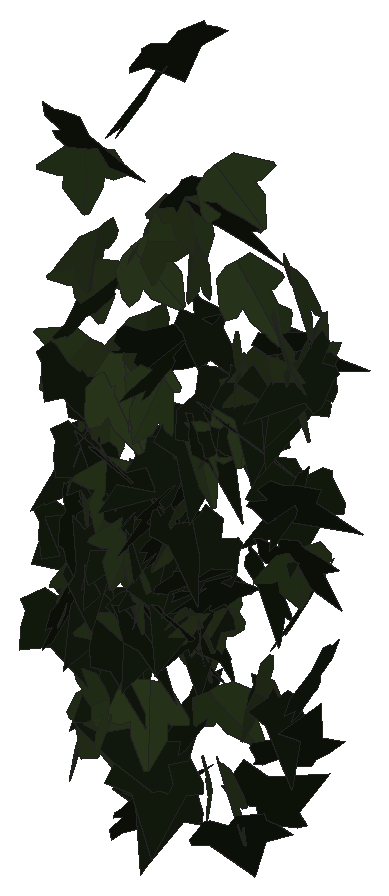
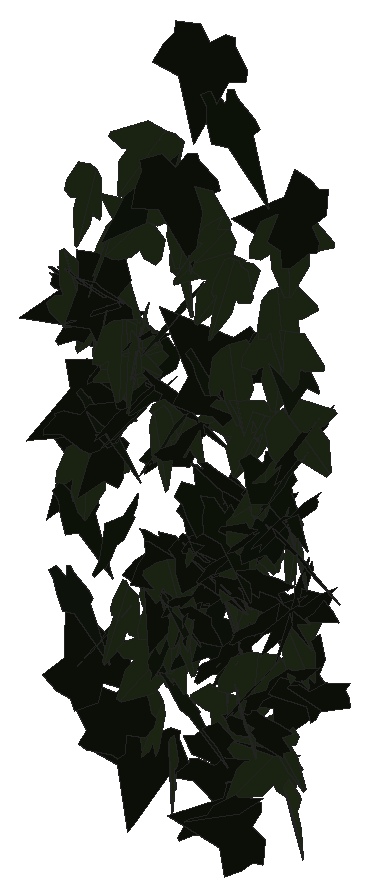
# SketchUp Ruby script. Lengths in inches.
U = 1.inch
M = Sketchup.active_model
def pt(a) = Geom::Point3d.new(a.map { |v| v * U })
def face(e, loops, mat)
  f = e.add_face(loops[0].map { |a| pt(a) })
  loops[1..].each { |l| e.add_face(l.map { |a| pt(a) }).erase! }
  f.material = f.back_material = mat if mat
  f
end
# faces: each face lists its corners as indices into pts; further lists are holes
def faces(e, pts, list, mat = nil) = list.each { |f| face(e, (f[0].is_a?(Array) ? f : [f]).map { |l| l.map { |i| pts[i] } }, mat) }
# xy, xz, yz: faces in a plane at the given z, y or x. An outline is a flat list of corners, or four numbers for a rectangle; further outlines are holes
def ring(l) = l.size == 4 ? [[l[0], l[1]], [l[2], l[1]], [l[2], l[3]], [l[0], l[3]]] : l.each_slice(2).to_a
def flat(e, list, mat, &to3) = list.each { |f| face(e, (f[0].is_a?(Array) ? f : [f]).map { |l| ring(l).map { |u, v| to3.(u, v) } }, mat) }
def xy(e, z, list, mat = nil) = flat(e, list, mat) { |x, y| [x, y, z] }
def xz(e, y, list, mat = nil) = flat(e, list, mat) { |x, z| [x, y, z] }
def yz(e, x, list, mat = nil) = flat(e, list, mat) { |y, z| [x, y, z] }
def lines(e, pts, list) = list.each { |a, b| e.add_line(pt(pts[a]), pt(pts[b])) }
# prism: a flat outline (further loops are holes) pulled along v
def prism(e, loops, v, mat = nil)
  f = face(e, loops, mat); d = Geom::Vector3d.new(v.map { |x| x * U })
  f.pushpull(f.normal.samedirection?(d) ? d.length : -d.length)
end
def box(e, o, s, mat = nil) = prism(e, [[o, [o[0] + s[0], o[1], o[2]], [o[0] + s[0], o[1] + s[1], o[2]], [o[0], o[1] + s[1], o[2]]]], [0, 0, s[2]], mat)
def at(x, y, z, deg = 0) = Geom::Transformation.translation(pt([x, y, z])) * Geom::Transformation.rotation(ORIGIN, Z_AXIS, deg.degrees)
def axes(o, x, y, z) = Geom::Transformation.new([*x, 0, *y, 0, *z, 0, *pt(o).to_a, 1])
def part(name) = M.definitions.add(name)
# library, detail: a bought-in or finely detailed component or shape, given as its bounding box
def library(name, o, s) = part(name).tap { |d| box(d.entities, o, s) }
def detail(e, o, s) = box(e.add_group.entities, o, s)
def put(e, d, t, mat = nil) = e.add_instance(d, t).tap { |i| i.material = mat if mat }
def group(e, t, mat = nil) = e.add_group.tap { |g| g.transformation = t; g.material = mat if mat }.entities
root = M.entities
M.materials.add("efeu1").color = [18, 25, 13]
M.materials.add("efeu2").color = [43, 57, 29]
c1 = part("ivyleaf_9")
p = [[1.54,2.16,1.25],[1.36,2.04,1.19],[-0.21,0.99,0.68],[-0.71,1.11,0.82],[-0.85,0.86,0.67],[-0.8,0.17,0.21],
  [-0.9,-0.01,0.1],[-0.67,-0.16,-0.02],[-0.08,-0.08,-0.05],[-0.03,-0.6,-0.4],[0.65,-0.88,-0.66],[0.83,-0.6,-0.49],
  [1.29,-0.42,-0.43],[1.8125,-0.07,-0.26],[1.21,0.44,0.15]]
faces(c1.entities,p,[[0,1,2,3,4,5,6,7,8,9,10,11,12,13,14]],"efeu1")
c2 = part("ivyleaf_10")
p = [[0,0.5,-0.03],[-0.0625,2.02,-0.43],[-0.19,2.01,-0.46],[-0.54,1.05,-0.29],[-0.52,0.625,-0.18],[-0.83,0.76,-0.28],
  [-1.16,0.64,-0.33],[-1.15,0.33,-0.24],[-0.77,-0.39,0.02],[-0.3,-0.51,0.16],[0.04,-0.48,0.23],[-0.02,2.01,-0.4375],
  [-0.06,2.01,-0.43],[0.04,-0.49,0.23],[0.67,-0.49,0.14],[1.38,0.36,-0.2],[1.375,0.51,-0.24],[0.81,0.65,-0.19],
  [0.62,0.59,-0.15],[0.6,1.09,-0.28],[0.5,1.23,-0.31]]
faces(c2.entities,p,[[0,1,2,3,4,5,6,7,8,9,10],[11,12,0,13,14,15,16,17,18,19,20]],"efeu2")
put(root,c1,axes([557.47,132.86,219.08],[0.60658,-0.54381,0.3875],[0.43826,-0.07075,-0.78533],[0.5038,0.71631,0.21662]))
put(root,c2,axes([552.82,132.8,225.43],[-0.73036,-0.58311,0.05549],[-0.04524,-0.03227,-0.93458],[0.584,-0.73175,-0.003]))
put(root,c2,axes([552.45,133.0625,219.47],[-0.53208,-0.47157,0.54848],[-0.39673,-0.37907,-0.71079],[0.60482,-0.66351,0.01627]))
put(root,c1,axes([554.42,132.75,215.25],[0.17808,-0.1101,0.87837],[-0.72136,0.5013,0.20908],[-0.51313,-0.74294,0.01091]))
put(root,c1,axes([555.13,132.63,228.52],[-0.57807,0.85894,-0.08509],[0.04941,-0.06931,-1.03534],[-0.86173,-0.58018,-0.00229]))
put(root,c1,axes([558.02,132.43,207.03],[0.55639,0.71118,-0.20448],[-0.13118,-0.15698,-0.90294],[-0.72827,0.57161,0.00643]))
put(root,c1,axes([559.49,132.37,217.54],[0.80214,0.25674,0.39294],[0.37203,0.12662,-0.8422],[-0.28619,0.88419,0.00651]))
put(root,c2,axes([557.59,132.82,208.22],[-0.69387,0.55552,-0.2453],[0.17651,-0.17188,-0.88856],[-0.58105,-0.7156,0.023]))
put(root,c2,axes([558.2,132.77,223.7],[0.71979,0.11011,0.65936],[0.63025,0.21122,-0.72329],[-0.22285,0.95301,0.08412]))
put(root,c2,axes([553.01,132.875,223.02],[-0.11838,-0.92552,-0.06851],[0.0011,0.06893,-0.93303],[0.92805,-0.11814,-0.00763]))
put(root,c1,axes([559.84,132.79,217.375],[-0.68343,0.5681,-0.01902],[0.01467,-0.01209,-0.88872],[-0.56823,-0.68359,-0.00008]))
put(root,c1,axes([552.0625,132.87,219.16],[0.36984,-0.75674,-0.35005],[-0.1662,0.30835,-0.84218],[0.81704,0.40527,-0.01286]))
put(root,c2,axes([560.07,132.7,224.38],[-0.82635,0.45852,0.04383],[-0.04635,0.00679,-0.9449],[-0.45827,-0.82749,0.01653]))
put(root,c1,axes([559.76,132.48,216.09],[0.90589,0.26652,-0.11191],[-0.10848,-0.02779,-0.94428],[-0.26794,0.91236,0.00393]))
put(root,c2,axes([556.46,133.02,218.1],[-0.81948,0.13079,-0.38359],[0.30779,-0.36207,-0.781],[-0.26365,-0.82921,0.28052]))
put(root,c2,axes([554.125,132.95,213.34],[-0.68982,0.39589,-0.33862],[0.22406,-0.28179,-0.7859],[-0.47031,-0.71492,0.12226]))
put(root,c2,axes([553.75,133.17,215.97],[-0.44081,-0.72991,0.3487],[-0.07843,-0.35668,-0.84575],[0.80511,-0.43438,0.10853]))
put(root,c1,axes([552.54,133.06,213.79],[-0.46389,-0.57428,-0.502],[0.31988,0.38692,-0.73822],[0.69245,-0.56347,0.00472]))
put(root,c1,axes([551.97,132.91,225.97],[0.66825,-0.28484,0.59393],[0.54404,-0.23831,-0.72641],[0.37135,0.8617,-0.00457]))
put(root,c2,axes([554.13,133.17,214.35],[-0.31867,-0.76691,0.29919],[-0.04618,-0.30366,-0.82757],[0.8219,-0.31441,0.0695]))
put(root,c1,axes([553.24,132.28,221.09],[0.00284,0.77291,0.49877],[-0.27206,0.47716,-0.73788],[-0.87872,-0.14523,0.23006]))
put(root,c2,axes([553.43,132.79,208.18],[-0.73599,-0.15467,-0.52759],[0.5255,0.06129,-0.75104],[0.16165,-0.90348,0.03937]))
put(root,c1,axes([557.26,132.54,225.55],[0.92495,0.13837,-0.00241],[-0.01675,0.09577,-0.93018],[-0.13737,0.91998,0.0972]))
put(root,c2,axes([554.96,132.5,223.23],[0.32845,0.66171,0.55842],[0.18607,0.52935,-0.73671],[-0.84561,0.3735,0.05479]))
put(root,c2,axes([559.94,132.89,215.67],[-0.43488,-0.76847,-0.11966],[0.04324,0.113,-0.88281],[0.77653,-0.43666,-0.01786]))
put(root,c1,axes([555.6,132.93,220.31],[-0.64013,0.64987,-0.10604],[0.00694,-0.14122,-0.90738],[-0.65842,-0.63329,0.09353]))
put(root,c2,axes([554.73,133,209.54],[0.93693,0.16638,0.14697],[0.14195,0.04108,-0.95147],[-0.17068,0.9475,0.01544]))
put(root,c1,axes([554.21,133.17,211.6],[0.49252,-0.69361,0.12402],[0.11232,-0.07209,-0.84926],[0.6956,0.50276,0.04932]))
put(root,c2,axes([554.95,132.99,219.03],[0.84963,-0.22571,-0.25975],[-0.23718,0.11724,-0.87766],[0.24933,0.88068,0.05027]))
put(root,c2,axes([559.14,132.85,221.28],[-0.91001,0.04005,0.01507],[-0.01501,0.00183,-0.91089],[-0.04008,-0.91014,-0.00117]))
put(root,c1,axes([555.9,132.51,230.2],[0.26752,0.91147,-0.06237],[-0.02542,-0.05754,-0.94988],[-0.91324,0.2686,0.00817]))
put(root,c2,axes([553.22,132.78,209.03],[0.49664,-0.30401,-0.70783],[-0.57736,0.41067,-0.58147],[0.51001,0.76094,0.03102]))
put(root,c2,axes([552.15,133.3,212.64],[0.19158,-0.8497,0.28444],[0.08541,-0.27223,-0.87074],[0.89196,0.20857,0.02229]))
put(root,c2,axes([556.31,132.91,225.16],[-0.82074,-0.4387,-0.06342],[0.05426,0.03301,-0.93062],[0.43992,-0.82252,-0.00353]))
put(root,c2,axes([559.48,132.75,222.6],[-0.51977,0.73445,0.16439],[-0.07068,0.15127,-0.89929],[-0.7493,-0.52374,-0.0292]))
put(root,c1,axes([554.99,133.31,207.55],[-0.51264,-0.63793,-0.33703],[0.23677,0.2418,-0.81781],[0.68153,-0.56385,0.0306]))
put(root,c1,axes([555.45,133.23,215.97],[-0.42253,0.57344,-0.53397],[0.13625,-0.54364,-0.69165],[-0.77162,-0.41001,0.17027]))
put(root,c1,axes([560.29,133.34,221.58],[-0.90128,0.04055,0.01997],[-0.02487,-0.11203,-0.89509],[-0.03774,-0.89452,0.11301]))
put(root,c1,axes([555.27,133.27,216.95],[-0.88487,0.07931,0.06994],[-0.07249,-0.02589,-0.88784],[-0.07698,-0.88725,0.03216]))
put(root,c2,axes([553.8,132.83,218.81],[0.55344,0.69538,0.34378],[0.23498,0.25218,-0.88838],[-0.73927,0.60074,-0.02501]))
put(root,c1,axes([555.15,133.2,207.66],[-0.30047,0.08024,0.86489],[-0.85799,0.11523,-0.30876],[-0.13539,-0.90832,0.03723]))
put(root,c1,axes([555.43,133.4,215.14],[0.2952,-0.80922,0.10957],[0.04443,-0.10042,-0.86136],[0.8154,0.29844,0.00727]))
put(root,c1,axes([559.91,133.48,221.53],[-0.7914,-0.35926,-0.22467],[0.25236,-0.01727,-0.86133],[0.34038,-0.8225,0.11622]))
put(root,c2,axes([555.5,132.48,224.08],[0.003,-0.3785,-0.84862],[0.30986,0.80046,-0.35592],[0.87602,-0.28184,0.1288]))
put(root,c2,axes([557.65,132.68,226.58],[0.46737,0.61433,0.53449],[0.19395,0.51455,-0.76101],[-0.79086,0.48923,0.12923]))
put(root,c1,axes([558.19,133.55,219.9],[-0.11464,-0.89674,0.0292],[-0.00024,-0.02941,-0.90403],[0.89721,-0.11459,0.00349]))
put(root,c1,axes([555.5,133.63,213.07],[-0.35716,-0.82388,0.04236],[0.00027,-0.04628,-0.89777],[0.82497,-0.35668,0.01863]))
put(root,c1,axes([553.42,133.36,210.83],[0.32268,-0.82099,-0.07439],[-0.00206,0.07908,-0.88172],[0.82436,0.32156,0.02692]))
put(root,c1,axes([558.76,133.6,210.63],[0.20915,-0.85335,0.22357],[0.09497,-0.20665,-0.87761],[0.87702,0.22588,0.04172]))
put(root,c2,axes([554.46,133.22,220.83],[-0.17141,-0.89668,-0.00621],[0.01263,0.00391,-0.91284],[0.89661,-0.17147,0.01167]))
put(root,c2,axes([555.4,133.72,214.92],[-0.11244,0.3847,-0.77795],[-0.0815,-0.78567,-0.37674],[-0.86404,0.02405,0.13678]))
put(root,c2,axes([558.76,132.67,211.3],[0.06453,-0.59585,-0.75032],[-0.0064,0.75173,-0.59753],[0.95811,0.04515,0.04654]))
put(root,c1,axes([552.05,132.42,211.17],[0.1319,0.30454,0.864],[0.24818,0.82839,-0.32988],[-0.88184,0.27868,0.03639]))
put(root,c1,axes([556.6875,132.99,226.08],[0.03785,0.86944,-0.33901],[-0.00626,-0.33905,-0.87023],[-0.93318,0.03754,-0.00791]))
put(root,c1,axes([554.51,132.99,220.05],[0.74729,0.66545,-0.25331],[0.16861,0.19138,1.00019],[0.69178,-0.7655,0.02986]))
put(root,c1,axes([556.42,133.03,221.75],[0.62156,-0.55565,-0.384],[-0.1649,0.38122,-0.81855],[0.65499,0.62327,0.15832]))
put(root,c2,axes([557.93,133.27,219.65],[0.50584,0.7239,-0.12618],[-0.05878,-0.11283,-0.88298],[-0.73246,0.50898,-0.01628]))
put(root,c2,axes([554.12,133.29,219.375],[0.7918,0.44741,-0.06621],[-0.05021,-0.04571,-0.90934],[-0.44949,0.79325,-0.01505]))
put(root,c1,axes([559.24,133.69,220.67],[-0.41567,-0.78854,-0.01827],[0.00399,0.01855,-0.89137],[0.78874,-0.41566,-0.00512]))
put(root,c1,axes([552.3125,133.33,216.57],[0.27475,-0.80355,-0.27842],[-0.02287,0.2855,-0.84656],[0.85011,0.26738,0.06721]))
put(root,c2,axes([552.73,133.17,221.86],[-0.79276,-0.45023,-0.02683],[0.01665,0.025,-0.91159],[0.45072,-0.79282,-0.01351]))
put(root,c1,axes([555.09,133.02,212.18],[0.89612,-0.10876,-0.00098],[-0.0009,0.00072,-0.9027],[0.10876,0.89612,0.00061]))
put(root,c2,axes([556.39,133.1,223.6875],[-0.68613,0.51321,0.36316],[-0.43244,0.00496,-0.82403],[-0.45637,-0.7763,0.23482]))
put(root,c1,axes([557.08,133.32,219.06],[-0.79787,0.2624,0.30518],[-0.28767,0.10211,-0.83989],[-0.28149,-0.84812,-0.0067]))
put(root,c1,axes([552.2,132.76,214.43],[0.32513,-0.07581,-0.86332],[-0.71821,0.49246,-0.31372],[0.48501,0.78007,0.11416]))
put(root,c1,axes([552.98,133.0625,216.24],[0.89559,-0.12999,-0.0139],[-0.01379,0.00174,-0.90498],[0.13,0.8957,-0.00026]))
put(root,c2,axes([557.19,133.08,210.3125],[-0.71086,-0.23411,-0.49745],[0.46955,0.16444,-0.74837],[0.28598,-0.8519,-0.00776]))
put(root,c2,axes([559.35,133.24,220.93],[-0.68691,0.54402,-0.25399],[0.20789,-0.14656,-0.87614],[-0.56325,-0.71755,-0.01361]))
put(root,c1,axes([556.04,133.77,217.85],[-0.13048,-0.88076,0.08198],[-0.00873,-0.08158,-0.89037],[0.88453,-0.13073,0.00331]))
put(root,c1,axes([552.27,133.5,217.93],[0.4561,-0.77566,-0.00192],[0.01766,0.01262,-0.89956],[0.77546,0.45593,0.02162]))
put(root,c1,axes([551.58,133.38,211.17],[-0.07751,-0.75806,-0.52624],[0.20412,0.50093,-0.75166],[0.89996,-0.17891,0.12516]))
put(root,c1,axes([558.36,133.26,207.48],[-0.0117,-0.16519,0.86926],[0.86455,-0.18713,-0.02392],[0.18829,0.84895,0.16387]))
put(root,c2,axes([554.68,132.99,223.42],[0.0315,-0.75243,-0.5322],[0.12535,0.53106,-0.7434],[0.91306,-0.04694,0.12042]))
put(root,c1,axes([555.47,133.52,216.48],[-0.57404,0.52944,-0.42353],[0.13641,-0.45341,-0.75168],[-0.66414,-0.55074,0.21168]))
put(root,c2,axes([558.35,133.41,220.4],[-0.1264,-0.90194,-0.0052],[0.00448,0.00462,-0.91075],[0.90195,-0.12642,0.0038]))
put(root,c2,axes([552.16,133.4,215.85],[-0.65587,0.57855,-0.19807],[0.0354,-0.25405,-0.85926],[-0.61049,-0.63629,0.16297]))
put(root,c1,axes([553.24,133.27,217.8125],[-0.47573,0.73736,-0.16871],[0.0171,-0.18877,-0.87325],[-0.75622,-0.46814,0.08639]))
put(root,c1,axes([556.41,133.12,213.74],[0.34982,0.70164,-0.38547],[-0.20828,-0.32641,-0.78316],[-0.77298,0.40548,0.03657]))
put(root,c1,axes([560.11,133.33,214.54],[-0.53911,0.67101,-0.2361],[0.15429,-0.17888,-0.86071],[-0.6944,-0.5607,-0.00795]))
put(root,c1,axes([555.36,133.59,213.96],[-0.85781,0.1344,-0.06234],[0.05082,-0.07711,-0.8656],[-0.13917,-0.85661,0.06814]))
put(root,c1,axes([556.37,133.48,212.5625],[-0.70701,0.44443,-0.24847],[0.18721,-0.16849,-0.83407],[-0.47351,-0.73021,0.04123]))
put(root,c1,axes([554.31,133.95,211.65],[-0.26299,-0.79086,0.24415],[-0.08866,-0.22778,-0.83336],[0.82292,-0.27729,-0.01176]))
put(root,c2,axes([552.1875,133.4375,207.5],[0.46432,-0.7013,-0.10271],[-0.05453,0.08708,-0.84108],[0.70668,0.4675,0.00258]))
put(root,c1,axes([555.4,133.54,214.78],[-0.29548,0.60973,-0.55694],[0.12928,-0.55007,-0.6708],[-0.81562,-0.30808,0.09544]))
put(root,c1,axes([556.38,133.67,217.9375],[0.42012,-0.78906,0.09861],[0.05516,-0.08234,-0.89388],[0.79328,0.42361,0.00993]))
put(root,c2,axes([552.04,133.54,216.3],[0.52172,-0.73387,0.02376],[0.01412,-0.01911,-0.90042],[0.73412,0.52191,0.00043]))
put(root,c2,axes([553.1,133.49,217.59],[0.01828,0.8674,-0.26461],[0.00516,-0.26476,-0.86753],[-0.90685,0.01598,-0.01027]))
put(root,c2,axes([554.3,133.53,212.99],[0.52773,-0.68683,-0.0084],[-0.00787,0.00454,-0.86615],[0.68684,0.52777,-0.00347]))
put(root,c1,axes([559.47,133.76,217.54],[-0.42417,-0.75561,-0.222],[0.11379,0.1907,-0.8665],[0.77928,-0.43913,0.00569]))
put(root,c2,axes([553.49,133.38,211.28],[-0.67821,-0.57029,-0.05161],[0.0356,0.03786,-0.88609],[0.57151,-0.67912,-0.00605]))
put(root,c1,axes([558.08,133.97,213.97],[0.23714,-0.66891,0.52929],[0.17067,-0.50105,-0.70968],[0.83574,0.29213,-0.00526]))
put(root,c1,axes([551.69,133.51,213.93],[0.27282,-0.7897,-0.36067],[0.03089,0.38665,-0.82322],[0.86761,0.23456,0.14273]))
put(root,c1,axes([552.375,133.66,216.01],[-0.86087,0.20506,-0.06305],[0.0559,-0.03734,-0.88465],[-0.20712,-0.86237,0.02331]))
put(root,c2,axes([557.85,132.94,220.67],[0.23391,-0.34468,-0.80439],[-0.161,0.80146,-0.39024],[0.86019,0.24373,0.1457]))
put(root,c1,axes([554.01,134.02,215.05],[-0.11401,-0.85111,0.18479],[0.01591,-0.18837,-0.85779],[0.87079,-0.10799,0.03987]))
put(root,c1,axes([556.48,133.84,214.61],[-0.84406,-0.19522,-0.12449],[0.13551,-0.03492,-0.86399],[0.18775,-0.85248,0.0639]))
put(root,c2,axes([556.02,133.4,212.21],[-0.67776,0.5337,-0.11149],[0.08344,-0.07425,-0.86265],[-0.5388,-0.68285,0.00666]))
put(root,c1,axes([559,133.51,209.08],[0.68242,0.57121,0.1933],[-0.14819,-0.12412,0.88994],[0.58454,-0.69833,-0.00005]))
put(root,c1,axes([554.45,133.94,215.48],[-0.48101,-0.73637,-0.10209],[0.09824,0.05757,-0.87811],[0.73689,-0.48835,0.05042]))
put(root,c1,axes([556.3,133.41,209.65],[-0.68908,0.58055,0.11951],[-0.09207,0.07621,-0.90103],[-0.58553,-0.6952,0.00103]))
put(root,c2,axes([556.49,133.55,212.23],[-0.44443,-0.77722,-0.01084],[0.00171,0.01151,-0.8953],[0.77729,-0.44441,-0.00422]))
put(root,c2,axes([555.81,133.6,212.3],[-0.06507,-0.86588,-0.03723],[-0.00407,0.03764,-0.8683],[0.86667,-0.06484,-0.00688]))
put(root,c1,axes([553.42,133.9,209.85],[-0.81513,-0.24427,-0.00506],[0.0047,0.00197,-0.85094],[0.24428,-0.81514,-0.00054]))
put(root,c1,axes([554.62,134.07,206.45],[-0.32464,-0.82684,0.07489],[-0.02001,-0.0726,-0.88826],[0.82999,-0.32516,0.00788]))
put(root,c1,axes([552.82,133.9,213.96],[-0.84381,-0.19726,-0.18221],[0.19112,-0.0191,-0.86443],[0.18864,-0.86305,0.06078]))
put(root,c2,axes([558.66,133.53,220],[0.18126,-0.00387,-0.88794],[-0.86825,0.18906,-0.17806],[0.186,0.88631,0.03411]))
put(root,c1,axes([556.49,133.13,213.36],[0.48056,0.72319,-0.05557],[-0.03499,-0.04346,-0.86828],[-0.72447,0.48181,0.00507]))
put(root,c2,axes([553.74,133.6875,210.37],[0.45201,-0.75716,-0.05301],[-0.04148,0.03696,-0.88166],[0.75788,0.45361,-0.01664]))
put(root,c1,axes([555.82,133.81,212.54],[-0.58669,-0.31593,-0.59243],[0.52915,0.26668,-0.66623],[0.41326,-0.78997,0.01202]))
put(root,c1,axes([552.76,134.23,213.43],[-0.29045,-0.77516,0.27355],[-0.00513,-0.28842,-0.82272],[0.822,-0.2757,0.09153]))
put(root,c2,axes([559.64,133.66,221.01],[-0.00207,-0.89541,0.09003],[-0.0021,0.09004,0.89541],[-0.89992,0.00185,-0.0023]))
put(root,c1,axes([554.1,132.97,205.79],[-0.01966,0.77556,-0.47178],[-0.00511,0.47179,0.77579],[0.90777,0.01945,-0.00585]))
put(root,c2,axes([558.01,133.41,220.16],[0.6287,-0.54632,-0.36655],[-0.06544,0.45257,-0.78676],[0.65463,0.56992,0.27339]))
put(root,c1,axes([553.54,134.06,214.42],[-0.75452,-0.4577,-0.00553],[0.00538,0.00179,-0.88249],[0.4577,-0.75454,0.00126]))
put(root,c2,axes([556.63,133.23,207.28],[0.31726,-0.39757,-0.70294],[-0.28552,0.65124,-0.4972],[0.75542,0.41312,0.1073]))
put(root,c1,axes([557.12,133.66,218.71],[0.48548,-0.72651,-0.21607],[0.00613,0.26034,-0.86161],[0.75794,0.46325,0.14537]))
put(root,c1,axes([557.59,133.91,218.55],[0.17901,-0.86299,-0.10728],[-0.00782,0.10792,-0.88124],[0.86959,0.17862,0.01415]))
put(root,c1,axes([554.62,133.3125,215.78],[-0.36292,0.81419,0.14316],[-0.07701,0.12237,-0.89119],[-0.82309,-0.37045,0.02026]))
put(root,c1,axes([560.12,133.56,211.87],[-0.59355,0.66654,-0.05058],[0.03442,-0.03708,-0.89252],[-0.66757,-0.59455,-0.00104]))
put(root,c1,axes([555.97,134.23,211.51],[0.57229,-0.37026,-0.54546],[0.4758,-0.26799,0.68112],[-0.45632,-0.74378,0.02612]))
put(root,c1,axes([558.76,133.22,221.42],[0.70764,0.14942,0.5741],[0.54537,0.18778,-0.7211],[-0.23343,0.89168,0.05566]))
put(root,c2,axes([556.7,133.73,218.09],[0.24432,-0.858,-0.093],[-0.00296,0.09583,-0.89181],[0.86302,0.24323,0.02328]))
put(root,c1,axes([552.3,134.26,211.43],[-0.35775,-0.74381,0.21767],[-0.09914,-0.19385,-0.82535],[0.76864,-0.3712,-0.00515]))
put(root,c2,axes([556.34,133.74,213.44],[-0.77957,-0.21492,0.37094],[-0.34057,-0.15707,-0.80676],[0.26038,-0.84891,0.05536]))
put(root,c2,axes([558.09,133.65,220.54],[-0.32921,-0.82957,-0.13957],[0.04625,0.1318,-0.89249],[0.83995,-0.3324,-0.00556]))
